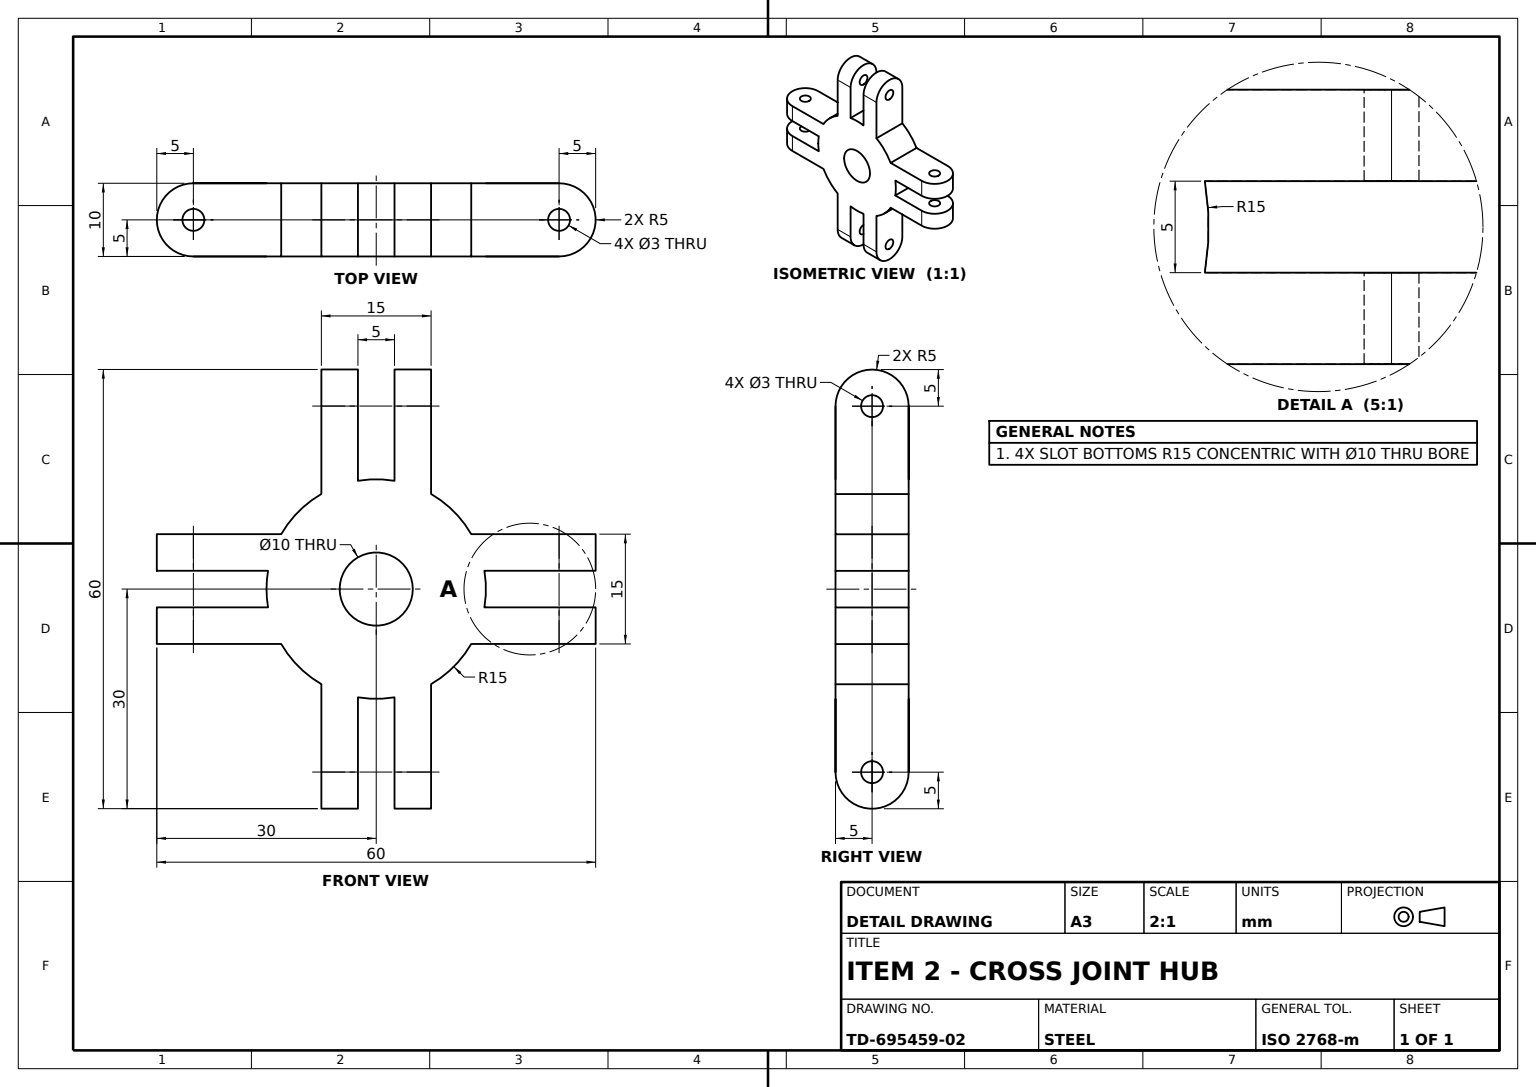
solid
v1 (2.5,30,0)
v2 (7.5,30,0)
e1 v1 v2 LINE
v3 (7.5,25,-5)
e2 v3 v2 CIRCLE(AX(P(7.5,25,0),D(1,0,0),D(0,1,0)),5)
v4 (2.5,25,-5)
e3 v4 v3 LINE
e4 v4 v1 CIRCLE(AX(P(2.5,25,0),D(1,0,0),D(0,1,0)),5)
face CYL(AX(P(-30,25,0),D(1,0,0),D(0,1,0)),5) [e1 -e2 -e3 e4]
v5 (-26.5,7.5,0)
v6 (-23.5,7.5,0)
e5 v5 v6 CIRCLE(AX(P(-25,7.5,0),D(0,1,0),D(-1,0,0)),1.5)
v7 (-23.5,2.5,0)
e6 v7 v6 LINE
v8 (-26.5,2.5,0)
e7 v8 v7 CIRCLE(AX(P(-25,2.5,0),D(0,1,0),D(-1,0,0)),1.5)
e8 v8 v5 LINE
face CYL(AX(P(-25,-30,0),D(0,1,0),D(-1,0,0)),1.5) rev [e5 -e6 -e7 e8]
v9 (-30,-7.5,0)
v10 (-30,-2.5,0)
e9 v9 v10 LINE
v11 (-25,-2.5,-5)
e10 v11 v10 CIRCLE(AX(P(-25,-2.5,0),D(0,1,0),D(-1,0,0)),5)
v12 (-25,-7.5,-5)
e11 v12 v11 LINE
e12 v12 v9 CIRCLE(AX(P(-25,-7.5,0),D(0,1,0),D(-1,0,0)),5)
face CYL(AX(P(-25,-30,0),D(0,1,0),D(-1,0,0)),5) [e9 -e10 -e11 e12]
v13 (2.5,-14.790199,5)
v14 (2.5,-14.790199,-5)
e13 v13 v14 LINE
v15 (-2.5,-14.790199,5)
e14 v15 v13 CIRCLE(AX(P(0,0,5),D(0,0,1),D(1,0,0)),15)
v16 (-2.5,-14.790199,-5)
e15 v15 v16 LINE
e16 v16 v14 CIRCLE(AX(P(0,0,-5),D(0,0,1),D(1,0,0)),15)
face CYL(AX(P(0,0,5),D(0,0,-1),D(-1,0,0)),15) [-e13 -e14 e15 e16]
v17 (23.5,-2.5,0)
v18 (26.5,-2.5,0)
e17 v17 v18 CIRCLE(AX(P(25,-2.5,0),D(0,-1,0),D(1,0,0)),1.5)
e18 v18 v17 CIRCLE(AX(P(25,-2.5,0),D(0,-1,0),D(1,0,0)),1.5)
v19 (25,-2.5,-5)
v20 (14.790199,-2.5,-5)
e19 v19 v20 LINE
v21 (14.790199,-2.5,5)
e20 v21 v20 LINE
v22 (25,-2.5,5)
e21 v22 v21 LINE
e22 v19 v22 CIRCLE(AX(P(25,-2.5,0),D(0,-1,0),D(1,0,0)),5)
face PLANE(AX(P(0,-2.5,5),D(0,-1,0),D(1,0,0))) rev [e17 e18] [e19 -e20 -e21 -e22]
v23 (-5,0,5)
v24 (-5,0,-5)
e23 v23 v24 LINE
v25 (5,0,-5)
e24 v25 v24 CIRCLE(AX(P(0,0,-5),D(0,0,1),D(1,0,0)),5)
v26 (5,0,5)
e25 v26 v25 LINE
e26 v26 v23 CIRCLE(AX(P(0,0,5),D(0,0,1),D(1,0,0)),5)
face CYL(AX(P(0,0,5),D(0,0,-1),D(-1,0,0)),5) rev [e23 -e24 -e25 e26]
v27 (2.5,14.790199,5)
v28 (2.5,14.790199,-5)
e27 v27 v28 LINE
v29 (-2.5,14.790199,-5)
e28 v28 v29 CIRCLE(AX(P(0,0,-5),D(0,0,1),D(1,0,0)),15)
v30 (-2.5,14.790199,5)
e29 v30 v29 LINE
e30 v27 v30 CIRCLE(AX(P(0,0,5),D(0,0,1),D(1,0,0)),15)
face CYL(AX(P(0,0,5),D(0,0,-1),D(-1,0,0)),15) [e27 e28 -e29 -e30]
v31 (-30,7.5,0)
v32 (-25,7.5,5)
e31 v31 v32 CIRCLE(AX(P(-25,7.5,0),D(0,1,0),D(-1,0,0)),5)
v33 (-12.990381,7.5,5)
e32 v32 v33 LINE
v34 (-12.990381,7.5,-5)
e33 v33 v34 LINE
v35 (-25,7.5,-5)
e34 v35 v34 LINE
e35 v35 v31 CIRCLE(AX(P(-25,7.5,0),D(0,1,0),D(-1,0,0)),5)
e36 v6 v5 CIRCLE(AX(P(-25,7.5,0),D(0,1,0),D(-1,0,0)),1.5)
face PLANE(AX(P(0,7.5,5),D(0,1,0),D(-1,0,0))) [e31 e32 e33 -e34 e35] [-e5 -e36]
v36 (7.5,-23.5,0)
v37 (7.5,-26.5,0)
e37 v36 v37 CIRCLE(AX(P(7.5,-25,0),D(1,0,0),D(0,1,0)),1.5)
v38 (2.5,-26.5,0)
e38 v38 v37 LINE
v39 (2.5,-23.5,0)
e39 v38 v39 CIRCLE(AX(P(2.5,-25,0),D(-1,0,0),D(0,-1,0)),1.5)
e40 v39 v36 LINE
face CYL(AX(P(-30,-25,0),D(1,0,0),D(0,1,0)),1.5) rev [e37 -e38 e39 e40]
v40 (-14.790199,2.5,-5)
v41 (-15,0,-5)
e41 v40 v41 CIRCLE(AX(P(0,0,-5),D(0,0,1),D(1,0,0)),15)
v42 (-25,2.5,-5)
e42 v42 v40 LINE
e43 v42 v35 LINE
v43 (-7.5,12.990381,-5)
e44 v43 v34 CIRCLE(AX(P(0,0,-5),D(0,0,1),D(1,0,0)),15)
v44 (-7.5,25,-5)
e45 v44 v43 LINE
v45 (-2.5,25,-5)
e46 v44 v45 LINE
e47 v45 v29 LINE
e48 v4 v28 LINE
v46 (7.5,12.990381,-5)
e49 v3 v46 LINE
v47 (12.990381,7.5,-5)
e50 v47 v46 CIRCLE(AX(P(0,0,-5),D(0,0,1),D(1,0,0)),15)
v48 (25,7.5,-5)
e51 v48 v47 LINE
v49 (25,2.5,-5)
e52 v49 v48 LINE
v50 (14.790199,2.5,-5)
e53 v49 v50 LINE
e54 v20 v50 CIRCLE(AX(P(0,0,-5),D(0,0,1),D(1,0,0)),15)
v51 (25,-7.5,-5)
e55 v51 v19 LINE
v52 (12.990381,-7.5,-5)
e56 v51 v52 LINE
v53 (7.5,-12.990381,-5)
e57 v53 v52 CIRCLE(AX(P(0,0,-5),D(0,0,1),D(1,0,0)),15)
v54 (7.5,-25,-5)
e58 v54 v53 LINE
v55 (2.5,-25,-5)
e59 v55 v54 LINE
e60 v55 v14 LINE
v56 (-2.5,-25,-5)
e61 v56 v16 LINE
v57 (-7.5,-25,-5)
e62 v57 v56 LINE
v58 (-7.5,-12.990381,-5)
e63 v57 v58 LINE
v59 (-12.990381,-7.5,-5)
e64 v59 v58 CIRCLE(AX(P(0,0,-5),D(0,0,1),D(1,0,0)),15)
e65 v12 v59 LINE
v60 (-14.790199,-2.5,-5)
e66 v11 v60 LINE
e67 v41 v60 CIRCLE(AX(P(0,0,-5),D(0,0,1),D(1,0,0)),15)
e68 v24 v25 CIRCLE(AX(P(0,0,-5),D(0,0,1),D(1,0,0)),5)
face PLANE(AX(P(0,0,-5),D(0,0,1),D(1,0,0))) rev [-e41 -e42 e43 e34 -e44 -e45 e46 e47 -e28 -e48 e3 e49 -e50 -e51 -e52 e53 -e54 -e19 -e55 e56 -e57 -e58 -e59 e60 -e16 -e61 -e62 e63 -e64 -e65 e11 e66 -e67] [e24 e68]
v61 (-7.5,-26.5,0)
v62 (-7.5,-23.5,0)
e69 v61 v62 CIRCLE(AX(P(-7.5,-25,0),D(-1,0,0),D(0,-1,0)),1.5)
e70 v62 v61 CIRCLE(AX(P(-7.5,-25,0),D(-1,0,0),D(0,-1,0)),1.5)
v63 (-7.5,-25,5)
v64 (-7.5,-12.990381,5)
e71 v63 v64 LINE
e72 v64 v58 LINE
e73 v57 v63 CIRCLE(AX(P(-7.5,-25,0),D(-1,0,0),D(0,-1,0)),5)
face PLANE(AX(P(-7.5,0,5),D(-1,0,0),D(0,-1,0))) [-e69 -e70] [e71 e72 -e63 e73]
v65 (25,7.5,5)
v66 (12.990381,7.5,5)
e74 v65 v66 LINE
e75 v65 v48 CIRCLE(AX(P(25,7.5,0),D(0,1,0),D(-1,0,0)),5)
e76 v66 v47 LINE
v67 (26.5,7.5,0)
v68 (23.5,7.5,0)
e77 v67 v68 CIRCLE(AX(P(25,7.5,0),D(0,1,0),D(-1,0,0)),1.5)
e78 v68 v67 CIRCLE(AX(P(25,7.5,0),D(0,1,0),D(-1,0,0)),1.5)
face PLANE(AX(P(0,7.5,5),D(0,-1,0),D(1,0,0))) rev [-e74 e75 e51 -e76] [-e77 -e78]
v69 (-7.5,12.990381,5)
e79 v69 v43 LINE
e80 v69 v33 CIRCLE(AX(P(0,0,5),D(0,0,1),D(1,0,0)),15)
face CYL(AX(P(0,0,5),D(0,0,-1),D(-1,0,0)),15) [e79 e44 -e33 -e80]
v70 (2.5,25,5)
e81 v1 v70 CIRCLE(AX(P(2.5,25,0),D(1,0,0),D(0,1,0)),5)
v71 (7.5,25,5)
e82 v70 v71 LINE
e83 v2 v71 CIRCLE(AX(P(7.5,25,0),D(1,0,0),D(0,1,0)),5)
face CYL(AX(P(-30,25,0),D(1,0,0),D(0,1,0)),5) [e81 e82 -e83 -e1]
v72 (12.990381,-7.5,5)
e84 v72 v52 LINE
v73 (7.5,-12.990381,5)
e85 v73 v72 CIRCLE(AX(P(0,0,5),D(0,0,1),D(1,0,0)),15)
e86 v73 v53 LINE
face CYL(AX(P(0,0,5),D(0,0,-1),D(-1,0,0)),15) [e57 -e84 -e85 e86]
v74 (25,-7.5,5)
e87 v51 v74 CIRCLE(AX(P(25,-7.5,0),D(0,-1,0),D(1,0,0)),5)
e88 v74 v72 LINE
v75 (26.5,-7.5,0)
v76 (23.5,-7.5,0)
e89 v75 v76 CIRCLE(AX(P(25,-7.5,0),D(0,-1,0),D(1,0,0)),1.5)
e90 v76 v75 CIRCLE(AX(P(25,-7.5,0),D(0,-1,0),D(1,0,0)),1.5)
face PLANE(AX(P(0,-7.5,5),D(0,-1,0),D(1,0,0))) [-e56 e87 e88 e84] [-e89 -e90]
v77 (-2.5,-23.5,0)
e91 v62 v77 LINE
v78 (-2.5,-26.5,0)
e92 v78 v77 CIRCLE(AX(P(-2.5,-25,0),D(-1,0,0),D(0,-1,0)),1.5)
e93 v61 v78 LINE
face CYL(AX(P(-30,-25,0),D(1,0,0),D(0,1,0)),1.5) rev [e91 -e92 -e93 e69]
e94 v75 v18 LINE
e95 v76 v17 LINE
face CYL(AX(P(25,-30,0),D(0,1,0),D(-1,0,0)),1.5) rev [e90 e94 -e17 -e95]
e96 v37 v36 CIRCLE(AX(P(7.5,-25,0),D(1,0,0),D(0,1,0)),1.5)
v79 (7.5,-25,5)
e97 v79 v73 LINE
e98 v79 v54 CIRCLE(AX(P(7.5,-25,0),D(1,0,0),D(0,1,0)),5)
face PLANE(AX(P(7.5,0,5),D(-1,0,0),D(0,-1,0))) rev [-e37 -e96] [-e97 e98 e58 -e86]
v80 (-30,2.5,0)
e99 v80 v31 LINE
e100 v42 v80 CIRCLE(AX(P(-25,2.5,0),D(0,1,0),D(-1,0,0)),5)
face CYL(AX(P(-25,-30,0),D(0,1,0),D(-1,0,0)),5) [e99 -e35 -e43 e100]
v81 (-12.990381,-7.5,5)
e101 v81 v59 LINE
e102 v81 v64 CIRCLE(AX(P(0,0,5),D(0,0,1),D(1,0,0)),15)
face CYL(AX(P(0,0,5),D(0,0,-1),D(-1,0,0)),15) [e101 e64 -e72 -e102]
v82 (2.5,26.5,0)
v83 (7.5,26.5,0)
e103 v82 v83 LINE
v84 (2.5,23.5,0)
e104 v84 v82 CIRCLE(AX(P(2.5,25,0),D(1,0,0),D(0,1,0)),1.5)
v85 (7.5,23.5,0)
e105 v84 v85 LINE
e106 v85 v83 CIRCLE(AX(P(7.5,25,0),D(1,0,0),D(0,1,0)),1.5)
face CYL(AX(P(-30,25,0),D(1,0,0),D(0,1,0)),1.5) rev [-e103 -e104 e105 e106]
v86 (-14.790199,2.5,5)
e107 v86 v40 LINE
v87 (-15,0,5)
e108 v87 v41 LINE
e109 v86 v87 CIRCLE(AX(P(0,0,5),D(0,0,1),D(1,0,0)),15)
face CYL(AX(P(0,0,5),D(0,0,-1),D(-1,0,0)),15) [e107 e41 -e108 -e109]
e110 v77 v78 CIRCLE(AX(P(-2.5,-25,0),D(-1,0,0),D(0,-1,0)),1.5)
v88 (-2.5,-25,5)
e111 v88 v15 LINE
e112 v56 v88 CIRCLE(AX(P(-2.5,-25,0),D(-1,0,0),D(0,-1,0)),5)
face PLANE(AX(P(-2.5,0,5),D(-1,0,0),D(0,-1,0))) rev [e110 e92] [e61 -e15 -e111 -e112]
v89 (-25,2.5,5)
e113 v80 v89 CIRCLE(AX(P(-25,2.5,0),D(0,1,0),D(-1,0,0)),5)
e114 v89 v32 LINE
face CYL(AX(P(-25,-30,0),D(0,1,0),D(-1,0,0)),5) [-e99 e113 e114 -e31]
v90 (14.790199,2.5,5)
e115 v90 v50 LINE
e116 v21 v90 CIRCLE(AX(P(0,0,5),D(0,0,1),D(1,0,0)),15)
face CYL(AX(P(0,0,5),D(0,0,-1),D(-1,0,0)),15) [e54 -e115 -e116 e20]
v91 (2.5,-25,5)
e117 v55 v91 CIRCLE(AX(P(2.5,-25,0),D(-1,0,0),D(0,-1,0)),5)
e118 v91 v13 LINE
e119 v39 v38 CIRCLE(AX(P(2.5,-25,0),D(-1,0,0),D(0,-1,0)),1.5)
face PLANE(AX(P(2.5,0,5),D(-1,0,0),D(0,-1,0))) [e117 e118 e13 -e60] [-e39 -e119]
v92 (-7.5,26.5,0)
v93 (-2.5,26.5,0)
e120 v92 v93 LINE
v94 (-2.5,23.5,0)
e121 v93 v94 CIRCLE(AX(P(-2.5,25,0),D(1,0,0),D(0,1,0)),1.5)
v95 (-7.5,23.5,0)
e122 v95 v94 LINE
e123 v92 v95 CIRCLE(AX(P(-7.5,25,0),D(1,0,0),D(0,1,0)),1.5)
face CYL(AX(P(-30,25,0),D(1,0,0),D(0,1,0)),1.5) rev [e120 e121 -e122 -e123]
face CYL(AX(P(-30,-25,0),D(1,0,0),D(0,1,0)),1.5) rev [e119 e38 e96 -e40]
v96 (-25,-7.5,5)
v97 (-25,-2.5,5)
e124 v96 v97 LINE
e125 v10 v97 CIRCLE(AX(P(-25,-2.5,0),D(0,1,0),D(-1,0,0)),5)
e126 v9 v96 CIRCLE(AX(P(-25,-7.5,0),D(0,1,0),D(-1,0,0)),5)
face CYL(AX(P(-25,-30,0),D(0,1,0),D(-1,0,0)),5) [e124 -e125 -e9 e126]
v98 (-26.5,-2.5,0)
v99 (-23.5,-2.5,0)
e127 v98 v99 CIRCLE(AX(P(-25,-2.5,0),D(0,1,0),D(-1,0,0)),1.5)
v100 (-23.5,-7.5,0)
e128 v100 v99 LINE
v101 (-26.5,-7.5,0)
e129 v101 v100 CIRCLE(AX(P(-25,-7.5,0),D(0,1,0),D(-1,0,0)),1.5)
e130 v101 v98 LINE
face CYL(AX(P(-25,-30,0),D(0,1,0),D(-1,0,0)),1.5) rev [e127 -e128 -e129 e130]
e131 v95 v92 CIRCLE(AX(P(-7.5,25,0),D(1,0,0),D(0,1,0)),1.5)
v102 (-7.5,30,0)
v103 (-7.5,25,5)
e132 v102 v103 CIRCLE(AX(P(-7.5,25,0),D(1,0,0),D(0,1,0)),5)
e133 v44 v102 CIRCLE(AX(P(-7.5,25,0),D(1,0,0),D(0,1,0)),5)
e134 v103 v69 LINE
face PLANE(AX(P(-7.5,0,5),D(1,0,0),D(0,1,0))) rev [e131 e123] [-e132 -e133 e45 -e79 -e134]
e135 v23 v26 CIRCLE(AX(P(0,0,5),D(0,0,1),D(1,0,0)),5)
e136 v63 v88 LINE
e137 v91 v79 LINE
e138 v74 v22 LINE
v104 (25,2.5,5)
e139 v104 v90 LINE
e140 v104 v65 LINE
v105 (7.5,12.990381,5)
e141 v66 v105 CIRCLE(AX(P(0,0,5),D(0,0,1),D(1,0,0)),15)
e142 v71 v105 LINE
e143 v70 v27 LINE
v106 (-2.5,25,5)
e144 v106 v30 LINE
e145 v103 v106 LINE
e146 v89 v86 LINE
v107 (-14.790199,-2.5,5)
e147 v87 v107 CIRCLE(AX(P(0,0,5),D(0,0,1),D(1,0,0)),15)
e148 v97 v107 LINE
e149 v96 v81 LINE
face PLANE(AX(P(0,0,5),D(0,0,1),D(1,0,0))) [-e135 -e26] [-e71 e136 e111 e14 -e118 e137 e97 e85 -e88 e138 e21 e116 -e139 e140 e74 e141 -e142 -e82 e143 e30 -e144 -e145 e134 e80 -e32 -e114 e146 e109 e147 -e148 -e124 e149 e102]
e150 v82 v84 CIRCLE(AX(P(2.5,25,0),D(1,0,0),D(0,1,0)),1.5)
face PLANE(AX(P(2.5,0,5),D(1,0,0),D(0,1,0))) rev [-e81 -e4 e48 -e27 -e143] [e150 e104]
v108 (23.5,2.5,0)
e151 v108 v68 LINE
v109 (26.5,2.5,0)
e152 v108 v109 CIRCLE(AX(P(25,2.5,0),D(0,-1,0),D(1,0,0)),1.5)
e153 v109 v67 LINE
face CYL(AX(P(25,-30,0),D(0,1,0),D(-1,0,0)),1.5) rev [-e151 e152 e153 e77]
face CYL(AX(P(-30,-25,0),D(1,0,0),D(0,1,0)),5) [e112 -e136 -e73 e62]
face CYL(AX(P(0,0,5),D(0,0,-1),D(-1,0,0)),5) rev [e135 e25 -e68 -e23]
e154 v107 v60 LINE
face CYL(AX(P(0,0,5),D(0,0,-1),D(-1,0,0)),15) [e67 -e154 -e147 e108]
e155 v100 v101 CIRCLE(AX(P(-25,-7.5,0),D(0,1,0),D(-1,0,0)),1.5)
face PLANE(AX(P(0,-7.5,5),D(0,1,0),D(-1,0,0))) rev [e129 e155] [-e12 e65 -e101 -e149 -e126]
e156 v49 v104 CIRCLE(AX(P(25,2.5,0),D(0,-1,0),D(1,0,0)),5)
face CYL(AX(P(25,-30,0),D(0,1,0),D(-1,0,0)),5) [-e156 e52 -e75 -e140]
e157 v109 v108 CIRCLE(AX(P(25,2.5,0),D(0,-1,0),D(1,0,0)),1.5)
face CYL(AX(P(25,-30,0),D(0,1,0),D(-1,0,0)),1.5) rev [e157 e151 e78 -e153]
e158 v99 v98 CIRCLE(AX(P(-25,-2.5,0),D(0,1,0),D(-1,0,0)),1.5)
face PLANE(AX(P(0,-2.5,5),D(0,1,0),D(-1,0,0))) [e148 e154 -e66 e10 e125] [-e127 -e158]
face CYL(AX(P(-25,-30,0),D(0,1,0),D(-1,0,0)),1.5) rev [e158 -e130 -e155 e128]
face PLANE(AX(P(0,2.5,5),D(0,-1,0),D(1,0,0))) [-e152 -e157] [e156 e139 e115 -e53]
v110 (-2.5,30,0)
e159 v110 v106 CIRCLE(AX(P(-2.5,25,0),D(1,0,0),D(0,1,0)),5)
e160 v102 v110 LINE
face CYL(AX(P(-30,25,0),D(1,0,0),D(0,1,0)),5) [-e159 -e160 e132 e145]
e161 v105 v46 LINE
face CYL(AX(P(0,0,5),D(0,0,-1),D(-1,0,0)),15) [-e141 e76 e50 -e161]
e162 v83 v85 CIRCLE(AX(P(7.5,25,0),D(1,0,0),D(0,1,0)),1.5)
face CYL(AX(P(-30,25,0),D(1,0,0),D(0,1,0)),1.5) rev [-e150 e103 e162 -e105]
face CYL(AX(P(25,-30,0),D(0,1,0),D(-1,0,0)),1.5) rev [e95 -e18 -e94 e89]
face PLANE(AX(P(7.5,0,5),D(1,0,0),D(0,1,0))) [e2 e83 e142 e161 -e49] [-e106 -e162]
face CYL(AX(P(-30,-25,0),D(1,0,0),D(0,1,0)),5) [e59 -e98 -e137 -e117]
face CYL(AX(P(-30,-25,0),D(1,0,0),D(0,1,0)),1.5) rev [-e110 -e91 e70 e93]
e163 v94 v93 CIRCLE(AX(P(-2.5,25,0),D(1,0,0),D(0,1,0)),1.5)
face CYL(AX(P(-30,25,0),D(1,0,0),D(0,1,0)),1.5) rev [-e120 -e131 e122 e163]
e164 v45 v110 CIRCLE(AX(P(-2.5,25,0),D(1,0,0),D(0,1,0)),5)
face PLANE(AX(P(-2.5,0,5),D(1,0,0),D(0,1,0))) [-e121 -e163] [-e47 e164 e159 e144 e29]
e165 v7 v8 CIRCLE(AX(P(-25,2.5,0),D(0,1,0),D(-1,0,0)),1.5)
face CYL(AX(P(-25,-30,0),D(0,1,0),D(-1,0,0)),1.5) rev [-e165 e6 e36 -e8]
face CYL(AX(P(25,-30,0),D(0,1,0),D(-1,0,0)),5) [-e138 -e87 e55 e22]
face CYL(AX(P(-30,25,0),D(1,0,0),D(0,1,0)),5) [e160 -e164 -e46 e133]
face PLANE(AX(P(0,2.5,5),D(0,1,0),D(-1,0,0))) rev [e165 e7] [-e107 -e146 -e113 -e100 e42]
